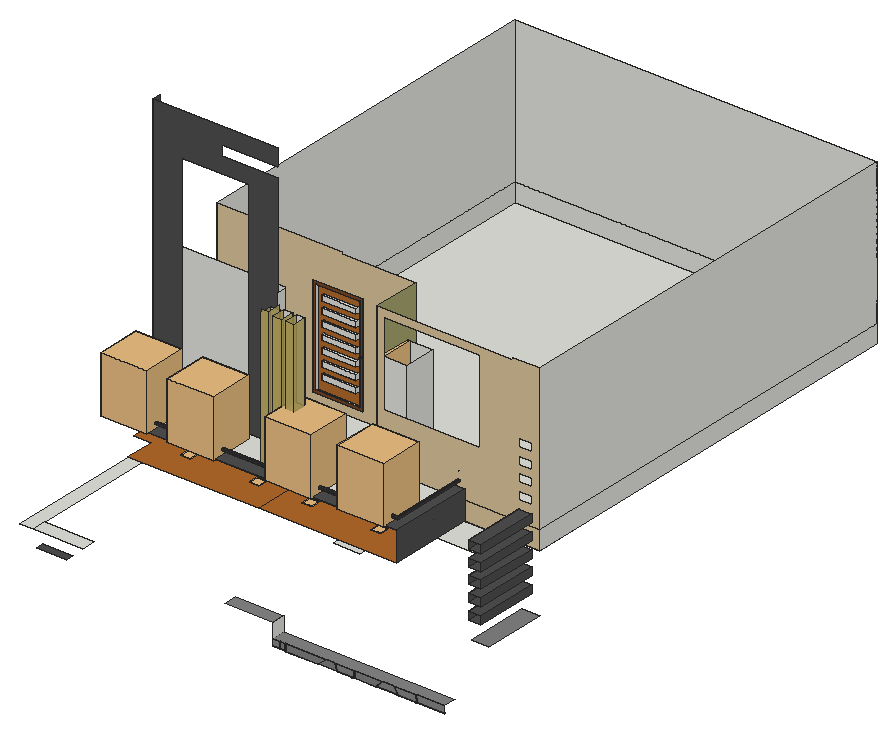
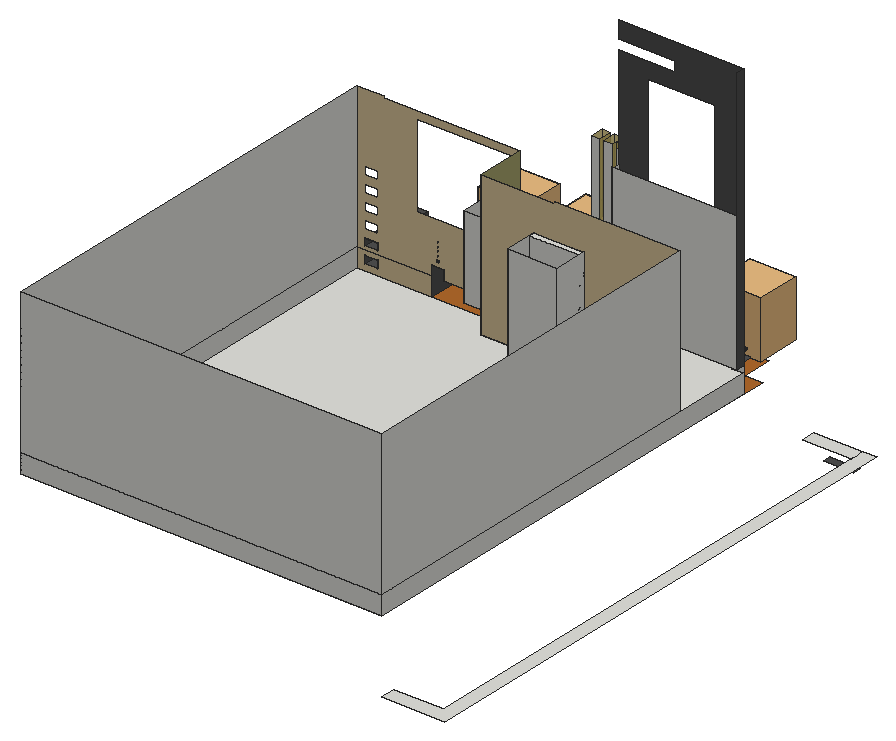
# SketchUp Ruby script. Lengths in inches.
U = 1.inch
M = Sketchup.active_model
def pt(a) = Geom::Point3d.new(a.map { |v| v * U })
def face(e, loops, mat)
  f = e.add_face(loops[0].map { |a| pt(a) })
  loops[1..].each { |l| e.add_face(l.map { |a| pt(a) }).erase! }
  f.material = f.back_material = mat if mat
  f
end
# faces: each face lists its corners as indices into pts; further lists are holes
def faces(e, pts, list, mat = nil) = list.each { |f| face(e, (f[0].is_a?(Array) ? f : [f]).map { |l| l.map { |i| pts[i] } }, mat) }
# xy, xz, yz: faces in a plane at the given z, y or x. An outline is a flat list of corners, or four numbers for a rectangle; further outlines are holes
def ring(l) = l.size == 4 ? [[l[0], l[1]], [l[2], l[1]], [l[2], l[3]], [l[0], l[3]]] : l.each_slice(2).to_a
def flat(e, list, mat, &to3) = list.each { |f| face(e, (f[0].is_a?(Array) ? f : [f]).map { |l| ring(l).map { |u, v| to3.(u, v) } }, mat) }
def xy(e, z, list, mat = nil) = flat(e, list, mat) { |x, y| [x, y, z] }
def xz(e, y, list, mat = nil) = flat(e, list, mat) { |x, z| [x, y, z] }
def yz(e, x, list, mat = nil) = flat(e, list, mat) { |y, z| [x, y, z] }
def lines(e, pts, list) = list.each { |a, b| e.add_line(pt(pts[a]), pt(pts[b])) }
# prism: a flat outline (further loops are holes) pulled along v
def prism(e, loops, v, mat = nil)
  f = face(e, loops, mat); d = Geom::Vector3d.new(v.map { |x| x * U })
  f.pushpull(f.normal.samedirection?(d) ? d.length : -d.length)
end
def box(e, o, s, mat = nil) = prism(e, [[o, [o[0] + s[0], o[1], o[2]], [o[0] + s[0], o[1] + s[1], o[2]], [o[0], o[1] + s[1], o[2]]]], [0, 0, s[2]], mat)
def at(x, y, z, deg = 0) = Geom::Transformation.translation(pt([x, y, z])) * Geom::Transformation.rotation(ORIGIN, Z_AXIS, deg.degrees)
def axes(o, x, y, z) = Geom::Transformation.new([*x, 0, *y, 0, *z, 0, *pt(o).to_a, 1])
def part(name) = M.definitions.add(name)
# library, detail: a bought-in or finely detailed component or shape, given as its bounding box
def library(name, o, s) = part(name).tap { |d| box(d.entities, o, s) }
def detail(e, o, s) = box(e.add_group.entities, o, s)
def put(e, d, t, mat = nil) = e.add_instance(d, t).tap { |i| i.material = mat if mat }
def group(e, t, mat = nil) = e.add_group.tap { |g| g.transformation = t; g.material = mat if mat }.entities
root = M.entities
M.materials.add("Generic").color = [129, 129, 129]
M.materials["Generic"].alpha = 0.97
M.materials.add("Generic\#1").color = [79, 79, 79]
M.materials.add("Generic\#2").color = [168, 165, 110]
M.materials.add("Generic\#3").color = [219, 197, 155]
M.materials.add("Generic\#6").color = [129, 129, 129]
M.materials.add("[Color M07]").color = [196, 178, 100]
M.materials["[Color M07]"].alpha = 0.86
M.materials.add("[Color M07]1").color = [58, 58, 58]
M.materials.add("[Wood Bamboo]").color = [177, 105, 43]
M.materials.add("[Wood Veneer 01]").color = [120, 70, 37]
c1 = library("Tlon Light 450 Ceiling 152 006",[-8.86,-8.86,-3.78],[17.72,17.72,3.56])
c2 = part("Group\#5")
xy(c2.entities,0,[[0,2.125,49.6875,7.875]])
xy(c2.entities,2.71,[[2.71,2.125,46.98,4.875]])
xy(c2.entities,13.9,[[8.49,2.125,42.99,4.875]])
xy(c2.entities,19.09,[[8.49,2.125,42.99,4.875]])
xy(c2.entities,25.71,[[8.49,2.125,42.99,4.875]])
xy(c2.entities,30.9,[[8.49,2.125,42.99,4.875]])
xy(c2.entities,37.52,[[8.49,2.125,42.99,4.875]])
xy(c2.entities,42.71,[[8.49,2.125,42.99,4.875]])
xy(c2.entities,49.34,[[8.49,2.125,42.99,4.875]])
xy(c2.entities,54.52,[[8.49,2.125,42.99,4.875]])
xy(c2.entities,61.15,[[8.49,2.125,42.99,4.875]])
xy(c2.entities,66.34,[[8.49,2.125,42.99,4.875]])
xy(c2.entities,72.96,[[8.49,2.125,42.99,4.875]])
xy(c2.entities,78.15,[[8.49,2.125,42.99,4.875]])
xy(c2.entities,84.77,[[8.49,2.125,42.99,4.875]])
xy(c2.entities,89.96,[[8.49,2.125,42.99,4.875]])
xy(c2.entities,97.73,[[2.71,2.125,46.98,4.875]])
xy(c2.entities,100.4375,[[0,2.125,49.6875,7.875]])
xz(c2.entities,0,[[48.27,47.74,48.43,47.76,48.58,47.82,48.71,47.92,48.8125,48.05,48.875,48.2,48.89,48.36,48.875,48.52,48.8125,48.67,48.71,48.8,48.58,48.9,48.43,48.97,48.27,48.99,48.11,48.97,47.96,48.9,47.83,48.8,47.73,48.67,47.67,48.52,47.64,48.36,47.67,48.2,47.73,48.05,47.83,47.92,47.96,47.82,48.11,47.76]])
xz(c2.entities,2.125,[[8.49,13.9,42.99,19.09],[8.49,25.71,42.99,30.9],[8.49,37.52,42.99,42.71],[48.27,47.74,48.11,47.76,47.96,47.82,47.83,47.92,47.73,48.05,47.67,48.2,47.64,48.36,47.67,48.52,47.73,48.67,47.83,48.8,47.96,48.9,48.11,48.97,48.27,48.99,48.43,48.97,48.58,48.9,48.71,48.8,48.8125,48.67,48.875,48.52,48.89,48.36,48.875,48.2,48.8125,48.05,48.71,47.92,48.58,47.82,48.43,47.76],[8.49,49.34,42.99,54.52],
  [8.49,61.15,42.99,66.34],[8.49,72.96,42.99,78.15],[8.49,84.77,42.99,89.96]])
xz(c2.entities,2.125,[[[0,0,49.6875,100.4375],[2.71,2.71,46.98,97.73],[48.27,47.74,48.11,47.76,47.96,47.82,47.83,47.92,47.73,48.05,47.67,48.2,47.64,48.36,47.67,48.52,47.73,48.67,47.83,48.8,47.96,48.9,48.11,48.97,48.27,48.99,48.43,48.97,48.58,48.9,48.71,48.8,48.8125,48.67,48.875,48.52,48.89,48.36,48.875,48.2,48.8125,48.05,48.71,47.92,48.58,47.82,48.43,47.76]]],"[Wood Veneer 01]")
xz(c2.entities,4.875,[[[2.71,2.71,46.98,97.73],[8.49,84.77,42.99,89.96],[8.49,72.96,42.99,78.15],[8.49,61.15,42.99,66.34],[8.49,49.34,42.99,54.52],[8.49,37.52,42.99,42.71],[8.49,25.71,42.99,30.9],[8.49,13.9,42.99,19.09]]],"[Wood Bamboo]")
xz(c2.entities,7.875,[[0,0,49.6875,100.4375]])
yz(c2.entities,0,[[2.125,0,7.875,100.4375]])
yz(c2.entities,2.71,[[2.125,2.71,4.875,97.73]])
yz(c2.entities,8.49,[[2.125,13.9,4.875,19.09],[2.125,25.71,4.875,30.9],[2.125,37.52,4.875,42.71],[2.125,49.34,4.875,54.52],[2.125,61.15,4.875,66.34],
  [2.125,72.96,4.875,78.15],[2.125,84.77,4.875,89.96]])
yz(c2.entities,42.99,[[2.125,13.9,4.875,19.09],[2.125,25.71,4.875,30.9],[2.125,37.52,4.875,42.71],[2.125,49.34,4.875,54.52],[2.125,61.15,4.875,66.34],
  [2.125,72.96,4.875,78.15],[2.125,84.77,4.875,89.96]])
yz(c2.entities,46.98,[[2.125,2.71,4.875,97.73]])
yz(c2.entities,49.6875,[[2.125,0,7.875,100.4375]])
p = [[48.11,2.125,47.76],[48.27,2.125,47.74],[48.27,0,47.74],[48.11,0,47.76],[48.43,2.125,47.76],[48.43,0,47.76],
  [47.83,2.125,47.92],[47.96,2.125,47.82],[47.96,0,47.82],[47.83,0,47.92],[48.58,2.125,47.82],[48.58,0,47.82],
  [48.71,2.125,47.92],[48.71,0,47.92],[47.73,2.125,48.05],[47.73,0,48.05],[48.8125,2.125,48.05],[48.8125,0,48.05],
  [47.67,2.125,48.2],[47.67,0,48.2],[48.875,2.125,48.2],[48.875,0,48.2],[47.64,2.125,48.36],[47.64,0,48.36],
  [48.89,2.125,48.36],[48.89,0,48.36],[47.67,2.125,48.52],[47.67,0,48.52],[48.875,2.125,48.52],[48.875,0,48.52],
  [47.73,2.125,48.67],[47.73,0,48.67],[48.8125,2.125,48.67],[48.8125,0,48.67],[47.83,2.125,48.8],[47.83,0,48.8],
  [48.71,2.125,48.8],[48.71,0,48.8],[47.96,2.125,48.9],[47.96,0,48.9],[48.58,2.125,48.9],[48.58,0,48.9],
  [48.11,2.125,48.97],[48.11,0,48.97],[48.43,2.125,48.97],[48.43,0,48.97],[48.27,2.125,48.99],[48.27,0,48.99],
  [48.27,2.125,48.36],[48.27,0,48.36]]
faces(c2.entities,p,[[0,1,2,3],[1,4,5,2],[6,7,8,9],[7,0,3,8],[4,10,11,5],[10,12,13,11],[14,6,9,15],[12,16,17,13],
  [18,14,15,19],[16,20,21,17],[22,18,19,23],[20,24,25,21],[26,22,23,27],[24,28,29,25],[30,26,27,31],[28,32,33,29],
  [34,30,31,35],[32,36,37,33],[38,34,35,39],[36,40,41,37],[42,38,39,43],[40,44,45,41],[46,42,43,47],[44,46,47,45]])
lines(c2.entities,p,[[48,49]])
c3 = library("Group3\#1",[-238.15,54.18,0],[46.4,43.96,56.68])
c4 = library("Group\#6",[0,0,0],[4.375,32.17,82.28])
xy(root,50.4375,[[264.86,28.58,271.42,29.64],[272.42,28.58,277.21,29.64],[346.31,28.58,367.77,28.77],[310.55,29.27,328.5625,30.14]])
xy(root,50.4375,[[278.21,28.58,278.21,29.64,310.55,29.64,310.55,29.02,309.55,29.02,309.55,28.58],[310.55,28.58,328.5625,29.27],[389.94,28.58,389.94,28.77,346.31,28.77,346.31,29.02,345.31,29.02,345.31,28.77,329.5625,28.77,329.5625,29.02,328.5625,29.02,328.5625,29.27,408.34,29.27,408.34,28.77,390.94,28.77,390.94,28.58],[329.5625,28.58,345.31,28.77],[368.77,28.58,388.94,28.77],
  [390.94,28.58,408.34,28.77],[409.34,28.58,435.86,29.27]],"Generic\#1")
xy(root,55.23,[[29.32,28.58,59.9,36.21]],"Generic\#1")
xy(root,56.8125,[[264.86,28.58,271.42,28.58,271.42,29.64,272.42,29.64,272.42,28.58,277.21,28.58,277.21,29.64,278.21,29.64,278.21,28.58,317.43,28.58,317.43,29.02,318.43,29.02,318.43,28.58,326.67,28.58,326.67,29.02,327.67,29.02,327.67,28.58,345.31,28.58,345.31,29.02,346.31,29.02,346.31,28.58,373.34,28.58,373.34,28.77,374.34,28.77,374.34,28.58,384.83,28.58,384.83,28.77,385.83,28.77,385.83,28.58,406.85,28.58,406.85,29.27,407.85,29.27,407.85,28.58,435.86,28.58,435.86,42.52,264.86,42.52]],"Generic")
xy(root,71.1875,[[13.36,28.58,26.8,28.58,26.8,550.64,75.86,550.64,75.86,565.96,13.36,565.96],[26.8,28.58,75.86,42.52]])
xy(root,71.1875,[[216.99,28.58,264.86,42.52]],"Generic")
xy(root,71.97,[[223.67,155.6,249.48,187.66]])
xy(root,85.23,[[418.23,84.21,435.86,146.83]],"Generic\#6")
xy(root,91.48,[[137.0625,194.96,186.75,227.77]])
xy(root,102.26,[[415.03,84.21,427.87,146.83]],"Generic\#1")
xy(root,110.19,[[415.03,84.21,427.87,146.83]],"Generic\#1")
xy(root,118.13,[[415.03,84.21,427.87,146.83]],"Generic\#1")
xy(root,119.1,[[286.0625,146.83,381.5625,188.08]])
xy(root,126.07,[[415.03,84.21,427.87,146.83]],"Generic\#1")
xy(root,134.01,[[415.03,84.21,427.87,146.83]],"Generic\#1")
xy(root,141.94,[[415.03,84.21,427.87,146.83]],"Generic\#1")
xy(root,144,[[223.67,146.83,223.67,194.96,75.86,194.96,75.86,565.96,435.86,565.96,435.86,146.83]])
xy(root,144,[[93.35,62.71,93.35,92.14,75.86,92.14,75.86,194.96,223.67,194.96,223.67,62.71],[223.67,62.71,361.3125,146.83]],"[Wood Bamboo]")
xy(root,149.88,[[415.03,84.21,427.87,146.83]],"Generic\#1")
xy(root,157.82,[[415.03,84.21,427.87,146.83]],"Generic\#1")
xy(root,162.4375,[[[87.41,76.77,87.41,115.77,75.86,115.77,75.86,194.96,273.73,194.96,273.73,146.83,349.0625,146.83,349.0625,76.77],[209.8,81.79,218.24,95.44],[222.49,81.79,230.92,95.44],[235.17,81.79,243.61,95.44]]])
xy(root,165.76,[[415.03,84.21,427.87,146.83]],"Generic\#1")
xy(root,169.0625,[[75.86,115.77,200.23,124.21]])
xy(root,171.1,[[171.75,194.96,221.4375,227.77]])
xy(root,172.625,[[75.86,62.71,75.86,115.77,87.41,115.77,87.41,76.77,349.0625,76.77,349.0625,146.83,361.3125,146.83,361.3125,62.71]],"Generic\#1")
xy(root,173.69,[[415.03,84.21,427.87,146.83]],"Generic\#1")
xy(root,176.51,[[273.73,152,299.55,184.0625]])
xy(root,177.11,[[80.31,70.4,80.31,115.77,82.18,115.77,82.18,72.28,354.41,72.28,354.41,146.83,356.29,146.83,356.29,70.4]])
xy(root,178.98,[[80.32,70.42,356.27,70.42,356.27,146.83,354.4,146.83,354.4,72.29,82.2,72.29,82.2,115.77,80.32,115.77]],"[Color M07]1")
xz(root,28.58,[[264.86,50.4375,271.42,56.8125],[272.42,50.4375,277.21,56.8125],[329.5625,50.4375,345.31,50.4375,345.31,56.8125,327.67,56.8125],[368.77,50.4375,388.94,50.4375,384.83,56.8125,374.34,56.8125],[389.94,50.4375,408.34,50.4375,406.85,56.8125,385.83,56.8125],
  [409.34,50.4375,435.86,50.4375,435.86,56.8125,407.85,56.8125]],"Generic")
xz(root,28.58,[[278.21,50.4375,309.55,50.4375,317.43,56.8125,278.21,56.8125],[310.55,50.4375,328.5625,50.4375,326.67,56.8125,318.43,56.8125],[346.31,50.4375,367.77,50.4375,373.34,56.8125,346.31,56.8125]],"Generic\#6")
xz(root,28.77,[[367.77,50.4375,368.77,50.4375,374.34,56.8125,373.34,56.8125],[388.94,50.4375,389.94,50.4375,385.83,56.8125,384.83,56.8125]],"Generic\#1")
xz(root,29.02,[[309.55,50.4375,310.55,50.4375,318.43,56.8125,317.43,56.8125],[328.5625,50.4375,329.5625,50.4375,327.67,56.8125,326.67,56.8125],[345.31,50.4375,346.31,56.8125]],"Generic\#1")
xz(root,76.77,[[87.41,162.4375,223.3,172.625],[223.3,162.4375,349.0625,172.625]])
xz(root,81.79,[[209.8,162.4375,218.24,162.4375,218.24,308.875,210.94,308.875,210.94,304.8125,209.8,304.8125],[222.49,162.4375,230.92,306.4375],[235.17,162.4375,243.61,306.4375]],"[Color M07]")
xz(root,95.44,[[209.8,162.4375,218.24,304.8125],[222.49,162.4375,230.92,306.4375],[235.17,162.4375,243.61,306.4375]])
xz(root,115.77,[[75.86,162.4375,87.41,169.0625],[75.86,169.0625,87.41,172.625],[80.31,177.11,80.32,178.98,82.2,178.98,82.18,177.11]])
xz(root,115.77,[[[87.41,169.0625,200.23,169.0625,200.23,407.6,144.48,407.6,144.48,417.1,200.23,417.1,200.23,434,75.86,434,75.86,172.625,87.41,172.625],[104.69,197.89,171.4,391.89],[80.31,194.11,80.32,195.98,82.2,195.98,82.18,194.11],[80.31,189.67,80.32,191.54,82.2,191.54,82.18,189.67],[80.31,185.61,80.32,187.48,82.2,187.48,82.18,185.61],[80.31,181.49,80.32,183.35,82.2,183.35,82.18,181.49],[80.31,177.11,80.32,178.98,82.2,178.98,82.18,177.11]]],"Generic\#1")
xz(root,124.21,[[75.86,169.0625,200.23,306.4375]])
xz(root,146.83,[[[361.3125,144,435.86,162.4375],[415.03,149.88,427.87,157.82]],[[273.73,162.4375,349.0625,162.4375,349.0625,172.625,361.3125,172.625,361.3125,162.4375,435.86,162.4375,435.86,306.4375,409.3,306.4375,409.3,304.8125,273.73,304.8125],[280.99,214.58,376.49,297.7],[415.03,165.76,427.87,173.69],[415.03,181.63,427.87,189.57],[415.03,197.51,427.87,205.44],[415.03,213.38,427.87,221.32],[415.03,229.26,427.87,237.19],[354.41,194.11,354.4,195.98,356.27,195.98,356.29,194.11],[354.41,189.67,354.4,191.54,356.27,191.54,356.29,189.67],[354.41,185.61,354.4,187.48,356.27,187.48,356.29,185.61],[354.41,181.49,354.4,183.35,356.27,183.35,356.29,181.49],[354.41,177.11,354.4,178.98,356.27,178.98,356.29,177.11]]],"Generic\#3")
xz(root,194.96,[[[75.86,162.4375,273.73,162.4375,273.73,304.8125,200.23,304.8125,200.23,306.4375,75.86,306.4375],[171.75,171.1,221.4375,271.54]]],"Generic\#3")
xz(root,227.77,[[171.75,171.1,221.4375,271.54]])
xz(root,565.96,[[75.86,144,435.86,162.4375],[75.86,162.4375,435.86,306.4375]])
yz(root,75.86,[[115.77,144,565.96,162.4375],[194.96,162.4375,565.96,306.4375]])
yz(root,75.86,[[115.77,169.0625,124.21,434]],"Generic\#1")
yz(root,87.41,[[76.77,162.4375,115.77,172.625]])
yz(root,171.75,[[194.96,171.1,227.77,271.54]])
yz(root,200.23,[[115.77,169.0625,124.21,304.8125]])
yz(root,209.8,[[81.79,162.4375,95.44,304.8125]],"[Color M07]")
yz(root,218.24,[[81.79,162.4375,95.44,308.875]],"[Color M07]")
yz(root,221.4375,[[194.96,171.1,227.77,271.54]])
yz(root,222.49,[[81.79,162.4375,95.44,306.4375]],"[Color M07]")
yz(root,230.92,[[81.79,162.4375,95.44,306.4375]],"[Color M07]")
yz(root,235.17,[[81.79,162.4375,95.44,306.4375]],"[Color M07]")
yz(root,243.61,[[81.79,162.4375,95.44,306.4375]],"[Color M07]")
yz(root,264.86,[[28.58,56.8125,42.52,71.1875]])
yz(root,271.42,[[28.58,50.4375,29.64,56.8125]],"Generic\#1")
yz(root,272.42,[[28.58,50.4375,29.64,56.8125]],"Generic\#1")
yz(root,273.73,[[[146.83,162.4375,194.96,304.8125],[152,176.51,184.0625,176.51,184.17,258.79,152.11,258.79]]],"Generic\#2")
yz(root,277.21,[[28.58,50.4375,29.64,56.8125]],"Generic\#1")
yz(root,278.21,[[28.58,50.4375,29.64,56.8125]],"Generic\#1")
yz(root,299.55,[[152,176.51,152.11,258.79,184.17,258.79,184.0625,176.51]])
yz(root,345.31,[[28.58,50.4375,29.02,56.8125]],"Generic\#1")
yz(root,346.31,[[28.58,50.4375,29.02,56.8125]],"Generic\#1")
yz(root,349.0625,[[76.77,162.4375,146.83,172.625]])
yz(root,361.3125,[[62.71,144,146.83,172.625]],"Generic\#1")
yz(root,415.03,[[84.21,102.26,146.83,110.19],[84.21,118.13,146.83,126.07],[84.21,134.01,146.83,141.94],[84.21,149.88,146.83,157.82],[84.21,165.76,146.83,173.69]],"Generic\#1")
yz(root,427.87,[[84.21,102.26,146.83,110.19],[84.21,118.13,146.83,126.07],[84.21,134.01,146.83,141.94],[84.21,149.88,146.83,157.82],[84.21,165.76,146.83,173.69]],"Generic\#1")
yz(root,435.86,[[146.83,144,565.96,162.4375],[146.83,162.4375,565.96,306.4375]])
p = [[317.43,28.58,56.8125],[309.55,28.58,50.4375],[309.55,29.02,50.4375],[317.43,29.02,56.8125],[310.55,28.58,50.4375],[318.43,28.58,56.8125],
  [318.43,29.02,56.8125],[310.55,29.02,50.4375],[326.67,28.58,56.8125],[328.5625,28.58,50.4375],[328.5625,29.02,50.4375],[326.67,29.02,56.8125],
  [329.5625,28.58,50.4375],[327.67,28.58,56.8125],[327.67,29.02,56.8125],[329.5625,29.02,50.4375],[329.5625,28.77,50.4375],[373.34,28.58,56.8125],
  [367.77,28.58,50.4375],[367.77,28.77,50.4375],[373.34,28.77,56.8125],[368.77,28.58,50.4375],[374.34,28.58,56.8125],[374.34,28.77,56.8125],
  [368.77,28.77,50.4375],[384.83,28.58,56.8125],[388.94,28.58,50.4375],[388.94,28.77,50.4375],[384.83,28.77,56.8125],[389.94,28.58,50.4375],
  [385.83,28.58,56.8125],[385.83,28.77,56.8125],[389.94,28.77,50.4375],[406.85,28.58,56.8125],[408.34,28.58,50.4375],[408.34,28.77,50.4375],
  [408.34,29.27,50.4375],[406.85,29.27,56.8125],[409.34,28.58,50.4375],[407.85,28.58,56.8125],[407.85,29.27,56.8125],[409.34,29.27,50.4375],
  [273.73,152,176.51],[273.73,152.11,258.79],[299.55,152.11,258.79],[299.55,152,176.51],[273.73,184.17,258.79],[273.73,184.0625,176.51],
  [299.55,184.0625,176.51],[299.55,184.17,258.79],[80.32,115.77,178.98],[80.31,115.77,177.11],[80.31,70.4,177.11],[80.32,70.42,178.98],
  [356.29,70.4,177.11],[356.27,70.42,178.98],[356.29,146.83,177.11],[356.27,146.83,178.98],[82.18,115.77,177.11],[82.2,115.77,178.98],
  [82.2,72.29,178.98],[82.18,72.28,177.11],[354.4,72.29,178.98],[354.41,72.28,177.11],[354.4,146.83,178.98],[354.41,146.83,177.11],
  [349.0625,107.96,162.4375],[361.3125,107.96,162.4375],[81.11,115.77,178.09],[81.11,71.21,178.09],[355.49,71.21,178.09],[355.49,146.83,178.09]]
faces(root,p,[[0,1,2,3],[8,9,10,11],[12,13,14,15,16],[17,18,19,20],[21,22,23,24],[25,26,27,28],[29,30,31,32],[33,34,35,36,37],
  [38,39,40,41]],"Generic\#1")
faces(root,p,[[4,5,6,7],[42,43,44,45],[46,47,48,49],[61,60,62,63]])
faces(root,p,[[50,51,52,53],[53,52,54,55],[55,54,56,57],[58,59,60,61],[63,62,64,65]],"[Color M07]1")
lines(root,p,[[66,67],[68,69],[69,70],[70,71]])
put(root,c1,axes([317.53,95.39,144.12],[0.532,0,0],[0,0.532,0],[0,0,0.532]))
put(root,c1,axes([249.16,95.39,144.12],[0.532,0,0],[0,0.532,0],[0,0,0.532]))
put(root,c1,axes([196.47,95.39,144.12],[0.532,0,0],[0,0.532,0],[0,0,0.532]))
put(root,c1,axes([128.09,95.39,144.12],[0.532,0,0],[0,0.532,0],[0,0,0.532]))
put(root,c2,at(171.75,192.83,171.1))
put(root,c3,at(304.72,7.53,171.52))
put(root,c3,at(371.15,7.53,171.52))
put(root,c3,at(468.03,7.53,171.52))
put(root,c3,at(540.4,7.53,171.52))
put(root,c4,at(272.42,152,176.51))
